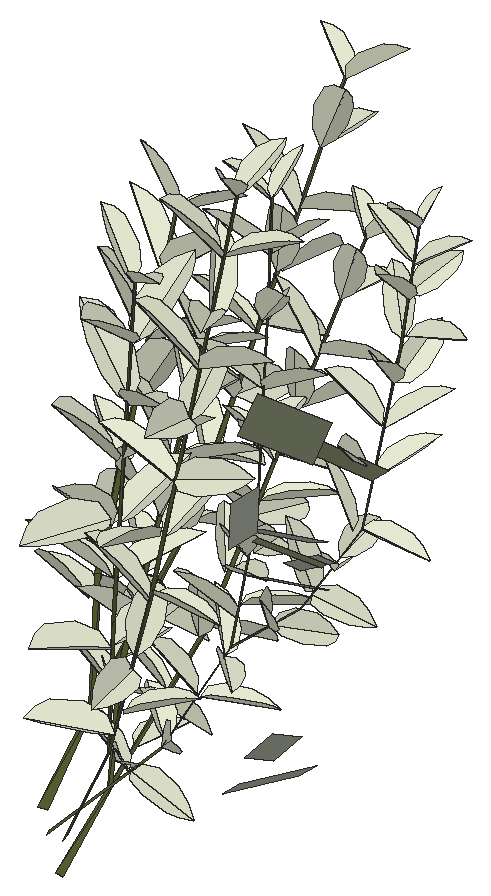
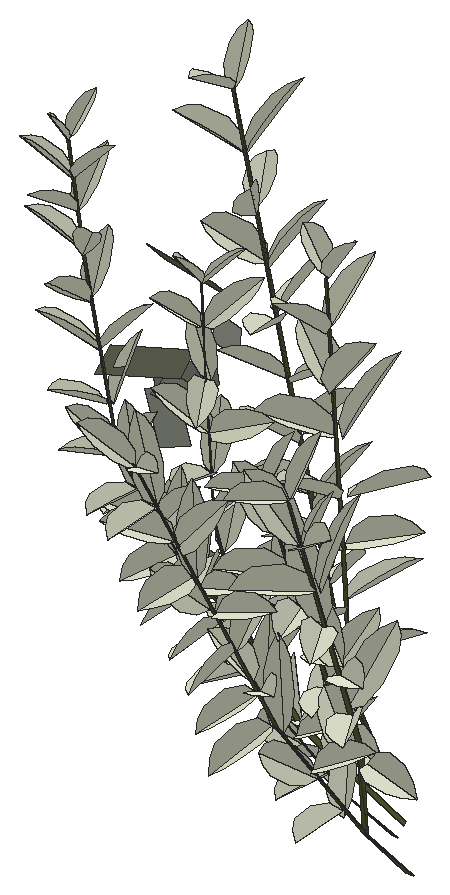
# SketchUp Ruby script. Lengths in inches.
U = 1.inch
M = Sketchup.active_model
def pt(a) = Geom::Point3d.new(a.map { |v| v * U })
def face(e, loops, mat)
  f = e.add_face(loops[0].map { |a| pt(a) })
  loops[1..].each { |l| e.add_face(l.map { |a| pt(a) }).erase! }
  f.material = f.back_material = mat if mat
  f
end
# faces: each face lists its corners as indices into pts; further lists are holes
def faces(e, pts, list, mat = nil) = list.each { |f| face(e, (f[0].is_a?(Array) ? f : [f]).map { |l| l.map { |i| pts[i] } }, mat) }
# xy, xz, yz: faces in a plane at the given z, y or x. An outline is a flat list of corners, or four numbers for a rectangle; further outlines are holes
def ring(l) = l.size == 4 ? [[l[0], l[1]], [l[2], l[1]], [l[2], l[3]], [l[0], l[3]]] : l.each_slice(2).to_a
def flat(e, list, mat, &to3) = list.each { |f| face(e, (f[0].is_a?(Array) ? f : [f]).map { |l| ring(l).map { |u, v| to3.(u, v) } }, mat) }
def xy(e, z, list, mat = nil) = flat(e, list, mat) { |x, y| [x, y, z] }
def xz(e, y, list, mat = nil) = flat(e, list, mat) { |x, z| [x, y, z] }
def yz(e, x, list, mat = nil) = flat(e, list, mat) { |y, z| [x, y, z] }
def lines(e, pts, list) = list.each { |a, b| e.add_line(pt(pts[a]), pt(pts[b])) }
# prism: a flat outline (further loops are holes) pulled along v
def prism(e, loops, v, mat = nil)
  f = face(e, loops, mat); d = Geom::Vector3d.new(v.map { |x| x * U })
  f.pushpull(f.normal.samedirection?(d) ? d.length : -d.length)
end
def box(e, o, s, mat = nil) = prism(e, [[o, [o[0] + s[0], o[1], o[2]], [o[0] + s[0], o[1] + s[1], o[2]], [o[0], o[1] + s[1], o[2]]]], [0, 0, s[2]], mat)
def at(x, y, z, deg = 0) = Geom::Transformation.translation(pt([x, y, z])) * Geom::Transformation.rotation(ORIGIN, Z_AXIS, deg.degrees)
def axes(o, x, y, z) = Geom::Transformation.new([*x, 0, *y, 0, *z, 0, *pt(o).to_a, 1])
def part(name) = M.definitions.add(name)
# library, detail: a bought-in or finely detailed component or shape, given as its bounding box
def library(name, o, s) = part(name).tap { |d| box(d.entities, o, s) }
def detail(e, o, s) = box(e.add_group.entities, o, s)
def put(e, d, t, mat = nil) = e.add_instance(d, t).tap { |i| i.material = mat if mat }
def group(e, t, mat = nil) = e.add_group.tap { |g| g.transformation = t; g.material = mat if mat }.entities
root = M.entities
M.materials.add("asdfasdf0165f6asdLeafVar1sfd015as60f1as6").color = [231, 235, 211]
M.materials.add("dw_stemssadfasdfa0sdf1s01d6w1").color = [90, 97, 50]
M.materials.add("viburnumblaasdfas0df1w06d").color = [98, 102, 84]
M.materials.add("viburnumbladsadfasdfad0w122").color = [125, 129, 119]
c1 = part("Component\#315")
p = [[0.25,0,0],[2.05,0.01,0.35],[1.81,4.2,1.66],[0,4.19,1.3125]]
faces(c1.entities,p,[[0,1,2,3]],"viburnumbladsadfasdfad0w122")
c2 = part("viburnumblad2")
put(c2.entities,c1,axes([-19.23,-4.49,-32.18],[83.35428,0,0],[0,79.38502,0],[0,0,83.35428]))
c3 = part("Component\#314")
p = [[0.14,0,0],[2.58,0.05,0.25],[2.44,5.11,2.64],[0,5.05,2.39]]
faces(c3.entities,p,[[0,1,2,3]],"viburnumblaasdfas0df1w06d")
c4 = part("viburnumblad1\#2")
put(c4.entities,c3,axes([-37.25,6.23,19.31],[75.98784,0,0],[0,65.50676,0],[0,0,75.98784]))
c5 = part("vdw_leaf\#3")
p = [[0,0,0],[-2.77,1.61,2.32],[-4.3125,6.1,4.5],[-3.97,13.49,6.09],[-2.47,18.57,6.3],[-0.2,22.73,5.75],
  [2.54,19.66,6.85],[4.3,15.93,7.09],[5.03,7.6,5.43],[3.32,1.76,2.74]]
faces(c5.entities,p,[[0,1,2,3,4,5],[0,5,6,7,8,9]],"asdfasdf0165f6asdLeafVar1sfd015as60f1as6")
c6 = part("dw_brancj_2\#2")
p = [[9.7,-0.22,29.95],[0.23,-1.96,0.34],[-0.05,1.51,0.11],[9.65,1.51,29.46],[18.64,-8.75,84.43],[18.96,-6.63,84.625],
  [1.53,6.02,63.68],[1.42,8.18,63.25],[-10.58,8.77,161.17],[-10.41,9.98,160.68],[26.34,-9.37,211.72],[26.57,-8.28,211.23]]
faces(c6.entities,p,[[0,1,2],[0,2,3],[4,0,3],[4,3,5],[6,0,3],[6,3,7],[8,6,7],[8,7,9],
  [10,4,5],[10,5,11]],"dw_stemssadfasdfa0sdf1s01d6w1")
c7 = part("vdw_branch2\#3")
put(c7.entities,c5,axes([19.53,-5.9,102.42],[1.12377,-0.50004,0],[0.46097,1.03596,0.47664],[-0.19377,-0.43548,1.13389]))
put(c7.entities,c5,axes([-5.89,6.52,109.44],[-1.07209,0.83679,0],[-0.77141,-0.98832,0.52702],[0.32427,0.41545,1.25373]))
put(c7.entities,c5,axes([-0.44,8.23,75.28],[0.88709,-0.9947,0],[0.92159,0.82189,0.33087],[-0.25219,-0.22491,1.26111]))
put(c7.entities,c5,axes([24.71,-8.97,190.81],[-0.82641,0.91101,0],[-0.83983,-0.76184,0.47664],[0.35303,0.32025,1.13389]))
put(c7.entities,c5,axes([-2.29,8.24,91.35],[1.24603,-0.47303,0],[0.43826,1.15445,0.33087],[-0.11993,-0.31592,1.26111]))
put(c7.entities,c5,axes([12.26,-3.11,37.92],[-0.64625,1.02205,0.22511],[-1.04383,-0.61044,-0.22511],[-0.07533,-0.30931,1.18809]))
put(c7.entities,c5,axes([26.17,-9.17,210.27],[-0.99452,-0.10453,0],[0.09636,-0.91681,0.38752],[-0.04051,0.38539,0.92186]))
put(c7.entities,c5,axes([-6.07,9.4,125.35],[-0.90214,-0.98107,0],[0.90896,-0.83583,0.33087],[-0.24874,0.22873,1.26111]))
put(c7.entities,c5,axes([-4.13,7.29,110.58],[0.44715,-1.078,0.64369],[1.05816,0.63649,0.33087],[-0.58725,0.40856,1.09216]))
put(c7.entities,c5,axes([23.91,-8.22,171.96],[0.62307,0.85009,-0.63406],[-0.71531,0.8798,0.47664],[0.78296,0.12729,0.94004]))
put(c7.entities,c6,at(-0.09,0.18,-0.25),"dw_stemssadfasdfa0sdf1s01d6w1")
put(c7.entities,c5,axes([23.34,-9.65,156.59],[-0.31364,-1.00782,0.58216],[1.10369,-0.17062,0.29925],[-0.17137,0.6239,0.98776]))
put(c7.entities,c5,axes([15.03,-3.37,58.83],[-1.05425,-0.00194,0.58442],[-0.14303,-1.11707,-0.26172],[0.55355,-0.3046,0.99755]))
put(c7.entities,c5,axes([-11.625,9.46,160.37],[0.36812,0.92978,0],[-0.85713,0.33936,0.38752],[0.3603,-0.14265,0.92186]))
put(c7.entities,c5,axes([21.32,-8.53,138.72],[1.21379,0.19904,0],[-0.19904,1.21379,0],[0,0,1.23]))
put(c7.entities,c5,axes([22.54,-9.2,141.43],[-1.02887,0.17955,0.60182],[-0.23387,-1.13057,-0.06253],[0.56696,-0.17376,1.02111]))
put(c7.entities,c5,axes([23.9,-8.82,173.84],[-1.14567,-0.37474,0],[0.35918,-1.0981,0.04438],[-0.01409,0.04308,1.17993]))
put(c7.entities,c5,axes([-7.84,8.92,143.59],[-1.26971,0.40522,0],[-0.37543,-1.17638,0.33087],[0.10274,0.32192,1.26111]))
put(c7.entities,c5,axes([19.77,-8.01,85.98],[-0.32405,-1.14591,0.18674],[1.10278,-0.32969,-0.10948],[0.15845,0.14442,1.16117]))
put(c7.entities,c5,axes([-0.62,5.76,76.34],[-0.08879,1.17576,-0.67771],[-1.34525,-0.16582,-0.11144],[-0.17897,0.66309,1.17383]))
put(c7.entities,c5,axes([20.49,-8.22,121.07],[0.39924,-0.78471,-0.8233],[1.08735,0.33121,0.2116],[0.09035,-0.83005,0.83495]))
put(c7.entities,c5,axes([15.15,-3.72,62.9],[1.16251,0.40128,-0.0211],[-0.39924,1.16074,0.07874],[0.0456,-0.06757,1.2273]))
put(c7.entities,c5,axes([20.72,-8.08,120.26],[-0.03693,1.2277,-0.06551],[-1.22944,-0.03698,0],[-0.00197,0.06548,1.22825]))
put(c7.entities,c5,axes([22.58,-8.36,155.57],[-0.56247,1.09386,0],[-1.00839,-0.51852,0.47664],[0.42389,0.21796,1.13389]))
put(c7.entities,c5,axes([3.97,3.13,57.96],[-1.09459,0.76041,0],[-0.72262,-1.0402,-0.1735],[-0.10109,-0.14552,1.29352]))
put(c7.entities,c5,axes([-10.8,9.06,160.75],[-0.66334,-0.72138,0],[0.66835,-0.61458,0.24329],[-0.1829,0.16818,0.92729]))
put(c7.entities,c5,axes([19.06,-9.3125,103.96],[-1.01345,0.25553,-0.60051],[-0.2265,-1.12952,-0.09839],[-0.59598,0.03076,1.01889]))
put(c7.entities,c5,axes([18.07,-6.2,81.7],[-0.56247,1.09386,0],[-1.00839,-0.51852,0.47664],[0.42389,0.21796,1.13389]))
put(c7.entities,c5,axes([12.95,-0.39,43.31],[0.13044,-1.19832,0],[1.11025,0.12085,0.29925],[-0.30382,-0.03307,1.14057]))
put(c7.entities,c5,axes([2.28,8.28,56.18],[1.32413,-0.31027,0],[0.30923,1.31968,-0.11144],[0.02542,0.1085,1.35543]))
put(c7.entities,c5,axes([-7.55,9.96,143.07],[1.34251,-0.21744,0],[0.20045,1.23761,0.52702],[-0.08426,-0.52024,1.25373]))
put(c7.entities,c5,axes([26.15,-8.25,210.66],[0.94661,-0.25364,0],[0.235,0.87703,0.24329],[-0.06431,-0.24,0.92729]))
put(c7.entities,c5,axes([-6.48,11.37,125.16],[0.64635,1.10315,0.46356],[-1.16569,0.46153,0.52702],[0.27017,-0.6478,1.16488]))
put(c7.entities,c5,axes([25.74,-8.35,191.28],[0.13044,-1.19832,0],[1.11025,0.12085,0.29925],[-0.30382,-0.03307,1.14057]))
put(c7.entities,c5,axes([-5.125,7.47,91.6],[-1.10024,0.63688,0.48318],[-0.78682,-1.00808,-0.46292],[0.14137,-0.65404,1.184]))
c8 = part("vdw_leaf\#2")
p = [[0,0,0],[-2.77,1.61,2.32],[-4.3125,6.1,4.5],[-3.97,13.49,6.09],[-2.47,18.57,6.3],[-0.2,22.73,5.75],
  [2.54,19.66,6.85],[4.3,15.93,7.09],[5.03,7.6,5.43],[3.32,1.76,2.74]]
faces(c8.entities,p,[[0,1,2,3,4,5],[0,5,6,7,8,9]],"asdfasdf0165f6asdLeafVar1sfd015as60f1as6")
c9 = part("dg_branch_1\#2")
p = [[46.12,1.57,35.62],[46,5.42,35.41],[0.14,1.79,0.05],[0.26,-2.0625,0.27],[74.05,2.99,75.8],[74.11,5.28,75.58],
  [103.46,0.47,94.74],[104.03,2.92,94.84],[81.14,16.92,120.46],[81.2,18.78,120.24],[130.47,-5.6875,130.27],[130.58,-3.66,129.85],
  [80.82,34.4375,191.22],[80.64,35.93,190.9],[148.49,-14.56,203.24],[148.9,-12.8125,203.11],[81.08,37.95,226.93],[81.4,39.1,227.03],
  [157.45,-18.19,250.77],[157.7,-17.01,250.41]]
faces(c9.entities,p,[[0,1,2,3],[4,0,1],[4,1,5],[6,4,5],[6,5,7],[8,4,5],[8,5,9],[10,6,7],
  [10,7,11],[12,8,9],[12,9,13],[14,10,11],[14,11,15],[16,12,13],[16,13,17],[18,14,15],
  [18,15,19]],"dw_stemssadfasdfa0sdf1s01d6w1")
c10 = part("vdw_branch1\#3")
put(c10.entities,c8,axes([120.69,-2.42,117.31],[1.12221,-0.24063,-0.65809],[0.19207,1.24776,-0.12871],[0.65778,0.01392,1.11658]))
put(c10.entities,c8,axes([81,38.9,226.05],[0.7888,-0.58155,0],[0.48308,0.65523,0.47],[-0.28484,-0.38635,0.83138]))
put(c10.entities,c8,axes([78.08,12.69,106.05],[-1.43826,-0.02353,-0.03177],[0.0088,-1.31777,0.57755],[-0.03854,0.57714,1.31741]))
put(c10.entities,c8,axes([130.18,-4.73,130.41],[-0.38031,-1.29044,-0.11242],[1.20662,-0.31032,-0.51987],[0.47109,-0.24694,1.24081]))
put(c10.entities,c8,axes([157.08,-17.89,249.93],[-0.91355,0.40674,0],[-0.37496,-0.84216,0.38752],[0.15762,0.35401,0.92186]))
put(c10.entities,c8,axes([90.64,3.03,86.49],[0.32514,-0.85045,-0.99675],[0.69523,0.98247,-0.61148],[1.11061,-0.36604,0.67459]))
put(c10.entities,c8,axes([80.15,28.42,160.95],[-0.16039,0.95636,-1.06292],[-1.41646,0.03966,0.24943],[0.19509,1.07422,0.93709]))
put(c10.entities,c8,axes([126.74,-5.45,129.22],[-0.59819,0.96152,-0.6841],[-0.85772,0.12575,0.92675],[0.75427,0.88089,0.57856]))
put(c10.entities,c8,axes([133.22,-6.12,150.66],[-0.93823,0.76985,0.59124],[-0.47726,-1.08188,0.65135],[0.84525,0.24366,1.02405]))
put(c10.entities,c8,axes([80.43,22.89,141.32],[-1.42571,-0.19312,0.01373],[0.18338,-1.31425,0.5561],[-0.0621,0.5528,1.32692]))
put(c10.entities,c8,axes([33.14,0.88,26.42],[-0.13338,1.31536,0.04876],[-1.04528,-0.13221,0.7073],[0.72315,0.03348,1.07497]))
put(c10.entities,c8,axes([152.63,-15.08,221.76],[-1.28188,0.41945,0.0579],[-0.3638,-1.18547,0.53367],[0.21665,0.49113,1.23869]))
put(c10.entities,c8,axes([80.05,28.28,160.33],[-0.46732,-1.26661,0.40679],[1.27397,-0.40257,0.21004],[-0.07408,0.44645,1.30501]))
put(c10.entities,c8,axes([153.95,-14.8,235.875],[0.39005,1.07743,0.20605],[-0.96443,0.25296,0.50293],[0.42961,-0.3464,0.99807]))
put(c10.entities,c8,axes([80.2,24.22,141.74],[1.33062,-0.46576,0.02628],[0.44746,1.2746,-0.06608],[-0.00197,0.0722,1.37936]))
put(c10.entities,c8,axes([145.48,-12.5,188.92],[-1.32952,0.16983,0.16138],[-0.09299,-1.2361,0.53471],[0.21503,0.51548,1.22904]))
put(c10.entities,c8,axes([139.64,-9.18,171.24],[0.05682,1.30088,0.23414],[-1.13176,-0.05343,0.57151],[0.58357,-0.22963,1.13417]))
put(c10.entities,c8,axes([70.95,4.35,71.98],[-1.1081,-0.41873,0.64752],[0.33675,-1.28259,-0.25313],[0.6937,-0.04625,1.15721]))
put(c10.entities,c8,axes([59.85,4.55,56.17],[-0.26797,1.24526,0.35754],[-0.9369,-0.41634,0.74783],[0.83377,-0.10389,0.98674]))
put(c10.entities,c8,axes([33.11,3.36,25.66],[-0.57817,-1.07968,-0.5679],[1.11554,-0.21356,-0.7297],[0.49375,-0.78178,0.98363]))
put(c10.entities,c9,at(-0.21,0.34,-0.17),"dw_stemssadfasdfa0sdf1s01d6w1")
put(c10.entities,c8,axes([80.91,19.01,122.53],[-0.84258,1.13222,-0.27981],[-1.15093,-0.75138,0.42537],[0.18861,0.47293,1.3457]))
put(c10.entities,c8,axes([119.8,-1.22,114.1],[-1.3235,-0.25012,0.09101],[0.25933,-1.31572,0.15537],[0.05991,0.1698,1.33794]))
put(c10.entities,c8,axes([46.29,5.1,38.04],[0.98937,0.73827,-0.47585],[-0.72359,1.03721,0.10473],[0.44068,0.18581,1.20453]))
put(c10.entities,c8,axes([81.1875,33.03,184.45],[1.33883,0.26986,0.35053],[-0.09581,1.22087,-0.57399],[-0.42216,0.53228,1.20262]))
put(c10.entities,c8,axes([80.16,36.28,206.98],[-0.83993,0.85737,-0.6234],[-1.05964,-0.65701,0.5241],[0.02941,0.81391,1.07976]))
put(c10.entities,c8,axes([154.86,-16.15,234.87],[0.02509,-1.15302,-0.28506],[1.1487,-0.04894,0.29908],[-0.30202,-0.28195,1.11384]))
put(c10.entities,c8,axes([108.77,-0.33,101.14],[-0.47691,-1.03266,-0.72709],[1.25395,-0.29455,-0.40416],[0.15052,-0.81814,1.06325]))
put(c10.entities,c8,axes([89.79,3.01,85.87],[-0.61344,0.75518,0.8965],[-0.17758,-1.01824,0.73622],[1.13385,0.22574,0.58569]))
put(c10.entities,c8,axes([81.56,20.31,123.29],[0.37259,-1.3435,0.21057],[1.29385,0.32364,-0.22445],[0.16906,0.25791,1.34638]))
put(c10.entities,c8,axes([46.45,1.82,36.74],[-0.77883,0.29892,1.0614],[0.19124,-1.24314,0.49044],[1.08598,0.43329,0.67484]))
put(c10.entities,c8,axes([71.37,4.02,72.32],[0.72905,0.81546,-0.74421],[-0.66805,0.98958,0.42988],[0.8391,0.14186,0.97745]))
put(c10.entities,c8,axes([136.59,-5.88,150.53],[0.85845,-0.99897,-0.12437],[0.96526,0.81273,0.13453],[-0.02572,-0.18182,1.28292]))
put(c10.entities,c8,axes([80.375,38.8,225.86],[-0.25178,0.96778,0],[-0.89216,-0.23211,0.38752],[0.37503,0.09757,0.92186]))
put(c10.entities,c8,axes([74.43,7.99,85.38],[-1.05703,0.91669,-0.33543],[-0.95806,-0.87958,0.61531],[0.18697,0.6754,1.25659]))
put(c10.entities,c8,axes([76.57,9.74,89.32],[0.63146,-1.21538,0.33508],[1.18148,0.49387,-0.43517],[0.26321,0.48577,1.26593]))
put(c10.entities,c8,axes([81.6875,36.97,207.4],[0.09422,-1.04424,0.38486],[1.01646,0.1939,0.27727],[-0.33299,0.33382,0.98727]))
put(c10.entities,c8,axes([157.29,-17.17,249.98],[0.50586,-0.50586,0],[0.38853,0.38853,0.41105],[-0.29684,-0.29684,0.56115]))
put(c10.entities,c8,axes([79.92,15.8,106.09],[1.03917,-0.29343,-0.90675],[-0.14587,1.22131,-0.5624],[0.92163,0.5191,0.88824]))
put(c10.entities,c8,axes([61.95,3.88,56.26],[0.41243,-1.28546,0],[1.17466,0.37688,-0.54831],[0.5221,0.16751,1.23363]))
put(c10.entities,c8,axes([151.99,-14.79,208.15],[-0.48571,-1.21723,-0.32393],[1.25386,-0.50033,0],[-0.12005,-0.30087,1.31056]))
put(c10.entities,c8,axes([108.44,0.62,102.22],[0.82183,0.96078,0.38967],[-0.62327,0.08618,1.10203],[0.79141,-0.88661,0.51693]))
put(c10.entities,c8,axes([145.6,-10.56,188.62],[1.03241,-0.02554,-0.82693],[0.3944,1.11584,0.45794],[0.70325,-0.61672,0.89706]))
put(c10.entities,c8,axes([78.59,32.3,183.89],[-1.12675,-0.42036,0.43987],[0.5899,-0.98149,0.57312],[0.14901,0.70693,1.05726]))
put(c10.entities,c8,axes([152.08,-13.42,223.37],[0.79993,-0.44251,-0.69938],[0.68456,0.82615,0.26026],[0.41048,-0.60953,0.85515]))
put(c10.entities,c8,axes([140.71,-8.74,170.55],[0.41903,-1.24177,-0.32393],[1.26224,0.33728,0.33986],[-0.23168,-0.40836,1.26573]))
put(c10.entities,c8,axes([149.25,-12.53,205.78],[1.24456,0.38285,0.23414],[-0.42999,1.04826,0.57151],[-0.02056,-0.62679,1.13417]))
put(root,c2,axes([1212,205.72,24.66],[0.00896,0.00518,0.00557],[-0.00512,0.01053,-0.00146],[-0.00544,-0.00118,0.00865]))
put(root,c2,axes([1214.8,207.75,11.73],[-0.00076,0.01192,-0.00361],[-0.00919,-0.00341,-0.00868],[-0.0089,0.00223,0.00792]))
put(root,c2,axes([1214.66,209.09,21.98],[0.00165,0.00828,-0.00613],[-0.01063,-0.00165,-0.00484],[-0.00434,0.00735,0.00651]))
put(root,c2,axes([1214.8125,210.23,22.93],[-0.00614,0.00518,-0.0082],[-0.00794,-0.00715,0.00088],[-0.00475,0.00709,0.00648]))
put(root,c2,axes([1212.97,208.02,11.875],[0.00484,0.0109,0.00393],[-0.00707,0.00614,-0.00813],[-0.00911,0.00107,0.00791]))
put(root,c4,axes([1215.43,209.05,29.1875],[0.00062,0.00927,0.00842],[-0.01215,0.00581,-0.0055],[-0.00687,-0.00679,0.00799]))
put(root,c7,axes([1198.9,209.13,1.63],[0.15791,0.02906,-0.03733],[-0.02958,0.1607,0],[0.02984,0.00549,0.19757]))
put(root,c2,axes([1213.24,210.61,23.46],[0.00132,0.00974,-0.00592],[-0.01063,-0.00165,-0.00484],[-0.00451,0.00633,0.00719]))
put(root,c2,axes([1213.39,209.91,22.14],[0.008,0.00859,-0.00017],[-0.00687,0.00594,-0.00742],[-0.00498,0.00541,0.0075]))
put(root,c4,axes([1215.1,213.98,25.58],[-0.00299,0.01151,-0.00453],[-0.01374,-0.0047,-0.00282],[-0.00346,0.0036,0.01051]))
put(root,c10,axes([1196.66,210.54,0.51],[0.11749,0.04939,0],[-0.04939,0.11749,0],[0,0,0.15683]))
put(root,c7,axes([1197.98,209.81,-1.1],[0.02729,0.1244,-0.09048],[-0.14364,0.03151,0],[0.01575,0.07182,0.15671]))
put(root,c7,axes([1193.88,213.63,-0.375],[0.0097,0.14118,-0.10053],[-0.16302,0.01121,0],[0.0056,0.08151,0.17413]))
